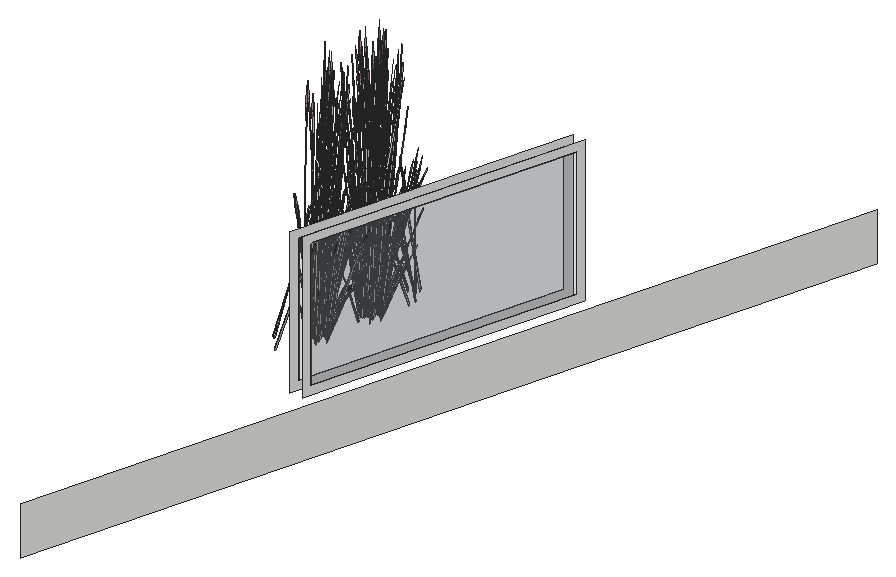
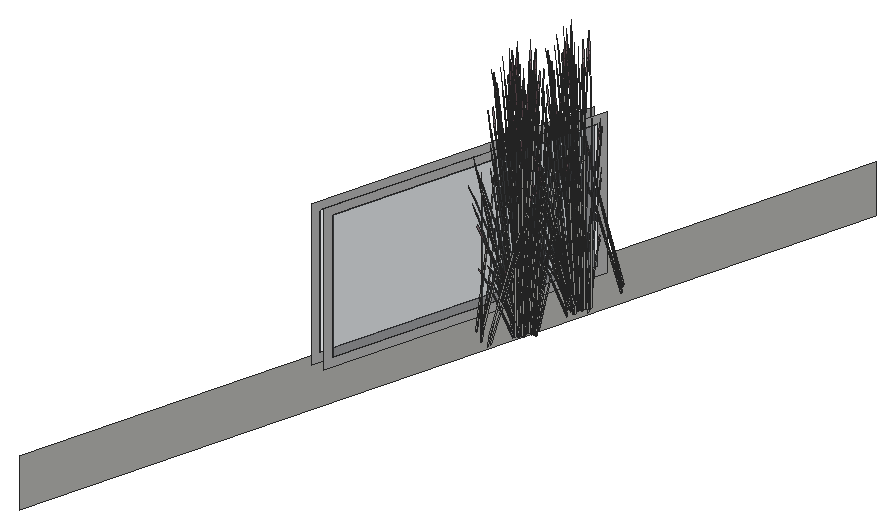
# SketchUp Ruby script. Lengths in inches.
U = 1.inch
M = Sketchup.active_model
def pt(a) = Geom::Point3d.new(a.map { |v| v * U })
def face(e, loops, mat)
  f = e.add_face(loops[0].map { |a| pt(a) })
  loops[1..].each { |l| e.add_face(l.map { |a| pt(a) }).erase! }
  f.material = f.back_material = mat if mat
  f
end
# faces: each face lists its corners as indices into pts; further lists are holes
def faces(e, pts, list, mat = nil) = list.each { |f| face(e, (f[0].is_a?(Array) ? f : [f]).map { |l| l.map { |i| pts[i] } }, mat) }
# xy, xz, yz: faces in a plane at the given z, y or x. An outline is a flat list of corners, or four numbers for a rectangle; further outlines are holes
def ring(l) = l.size == 4 ? [[l[0], l[1]], [l[2], l[1]], [l[2], l[3]], [l[0], l[3]]] : l.each_slice(2).to_a
def flat(e, list, mat, &to3) = list.each { |f| face(e, (f[0].is_a?(Array) ? f : [f]).map { |l| ring(l).map { |u, v| to3.(u, v) } }, mat) }
def xy(e, z, list, mat = nil) = flat(e, list, mat) { |x, y| [x, y, z] }
def xz(e, y, list, mat = nil) = flat(e, list, mat) { |x, z| [x, y, z] }
def yz(e, x, list, mat = nil) = flat(e, list, mat) { |y, z| [x, y, z] }
def lines(e, pts, list) = list.each { |a, b| e.add_line(pt(pts[a]), pt(pts[b])) }
# prism: a flat outline (further loops are holes) pulled along v
def prism(e, loops, v, mat = nil)
  f = face(e, loops, mat); d = Geom::Vector3d.new(v.map { |x| x * U })
  f.pushpull(f.normal.samedirection?(d) ? d.length : -d.length)
end
def box(e, o, s, mat = nil) = prism(e, [[o, [o[0] + s[0], o[1], o[2]], [o[0] + s[0], o[1] + s[1], o[2]], [o[0], o[1] + s[1], o[2]]]], [0, 0, s[2]], mat)
def at(x, y, z, deg = 0) = Geom::Transformation.translation(pt([x, y, z])) * Geom::Transformation.rotation(ORIGIN, Z_AXIS, deg.degrees)
def axes(o, x, y, z) = Geom::Transformation.new([*x, 0, *y, 0, *z, 0, *pt(o).to_a, 1])
def part(name) = M.definitions.add(name)
# library, detail: a bought-in or finely detailed component or shape, given as its bounding box
def library(name, o, s) = part(name).tap { |d| box(d.entities, o, s) }
def detail(e, o, s) = box(e.add_group.entities, o, s)
def put(e, d, t, mat = nil) = e.add_instance(d, t).tap { |i| i.material = mat if mat }
def group(e, t, mat = nil) = e.add_group.tap { |g| g.transformation = t; g.material = mat if mat }.entities
root = M.entities
M.materials.add("Glass_Basic_01").color = [105, 113, 122]
M.materials["Glass_Basic_01"].alpha = 0.25
M.materials.add("LightPink_Translucent").color = [144, 107, 117]
M.materials["LightPink_Translucent"].alpha = 0.75
M.materials.add("M01_Silver_Fog").color = [224, 224, 224]
c1 = part("blade")
p = [[2.15,0.21,22],[0,0.17,0],[0.09,0.45,0],[2.18,0.31,22],[2.29,0.31,22],[0.38,0.45,0],
  [2.48,0.24,33],[2.49,0.24,33],[2.48,0.22,33]]
faces(c1.entities,p,[[0,1,2,3],[4,5,2,3],[6,3,4,7],[8,0,3,6]])
c2 = part("seeds")
p = [[0.3,-0.1,1.38],[-0.01,-0.03,1.59],[-0.01,-0.03,0.03],[0.14,-0.07,-0.07],[0.29,-0.03,3],[0.15,0.01,3.11]]
faces(c2.entities,p,[[0,1,2,3],[1,0,4,5]],"LightPink_Translucent")
c3 = part("blade with seeds")
put(c3.entities,c1,at(0,0,0))
put(c3.entities,c2,axes([2.4,0.25,30.99],[1.5799,-0.05474,1.17369],[-0.12525,1.92788,0.29478],[-0.07173,-0.02425,1.56792]))
p = [[364.95,435.42,522],[307.76,240,522],[307.76,240,510.01],[307.76,240,510],[364.95,435.42,510],[321.22,307.35,558],
  [340.07,371.78,558],[340.07,371.78,522],[321.22,307.35,522],[339.51,369.86,524],[339.51,369.86,556],[321.78,309.27,556],
  [321.78,309.27,524],[343.2,371.78,558],[324.34,307.35,558],[324.34,307.35,522],[343.2,371.78,522],[324.9,309.27,524],
  [324.9,309.27,556],[342.64,369.86,556],[342.64,369.86,524]]
faces(root,p,[[0,1,2,3,4]])
faces(root,p,[[[5,6,7,8],[9,10,11,12]],[[13,14,15,16],[17,18,19,20]]],"M01_Silver_Fog")
faces(root,p,[[10,9,12,11],[18,17,20,19]],"Glass_Basic_01")
put(root,c3,axes([312.83,325.4,524.43],[0.56613,0.26102,0.24065],[-0.27246,0.54236,0.50002],[0,-0.12502,1.60543]))
put(root,c3,axes([313.73,325.53,524.29],[0,0.62282,-0.05637],[-0.62828,0,0],[0,0.01957,1.79368]))
put(root,c3,axes([310.27,315.96,526.53],[0.28589,0.33718,-0.35414],[-0.32644,0.31919,0.4572],[0.16586,0.04856,0.87481]))
put(root,c3,axes([312.65,325.04,524.72],[-0.54562,0.03324,0.44739],[-0.04934,-0.55185,-0.21531],[0.09768,-0.05593,1.43643]))
put(root,c3,axes([314.99,340.47,524.48],[0.47024,0.26927,0.49651],[-0.28107,0.48284,0],[-0.1071,-0.06133,1.57504]))
put(root,c3,axes([312.4,324.09,524.47],[-0.14515,0.53522,0.17642],[-0.53115,-0.15146,0.35086],[0.09175,-0.00261,1.60407]))
put(root,c3,axes([313.43,326.74,524.29],[0.21845,0.61869,-0.06012],[-0.62418,0.21679,0],[0.00763,0.02161,1.72173]))
put(root,c3,axes([315.4375,339.49,524.4375],[0.13317,-0.63814,-0.23429],[0.63143,0.11124,0.51271],[-0.11033,-0.08813,1.5644]))
put(root,c3,axes([315.67,339.64,524.62],[-0.09693,0.48062,0.1448],[-0.47357,-0.08343,-0.41347],[-0.08619,-0.04935,1.26744]))
put(root,c3,axes([316.61,340.98,524.02],[-0.47024,0.26927,-0.49651],[-0.28107,-0.48284,0],[-0.1071,0.06133,1.57504]))
put(root,c3,axes([313.82,338.29,524.02],[0,-0.53854,-0.49651],[0.56215,0,0],[0,-0.12266,1.57504]))
put(root,c3,axes([314.07,338.79,524.48],[0,0.53854,0.49651],[-0.56215,0,0],[0,-0.12266,1.57504]))
put(root,c3,axes([316.64,340.83,524.19],[-0.31023,-0.54153,-0.05142],[0.52557,-0.30095,0.51607],[-0.12951,0.05156,1.6363]))
put(root,c3,axes([312.14,323.43,524.375],[-0.31414,-0.53965,0],[0.52557,-0.30095,-0.51607],[0.1197,-0.06854,1.63711]))
put(root,c3,axes([312.71,327.49,526.98],[0.23981,0.43789,-0.71045],[-0.49365,0.24404,0.08574],[0.05608,0.21158,1.00501]))
put(root,c3,axes([315.24,325.93,524.2],[-0.62797,-0.00431,-0.04976],[0,-0.6019,0.49943],[-0.01973,0.13702,1.58352]))
put(root,c3,axes([314,324.12,524.47],[-0.53992,0.14294,0.17642],[-0.13332,-0.53195,0.35086],[0.04815,0.07751,1.60407]))
put(root,c3,axes([316.5,340.76,524.03],[-0.46876,-0.13325,-0.30978],[0.11803,-0.46926,0.30978],[-0.0945,0.05411,1.38974]))
put(root,c3,axes([313.45,322.125,524.77],[0.06446,0.31404,1.1486],[-0.35756,-0.17393,0.84392],[0.03848,-0.1608,0.25299]))
put(root,c3,axes([315.29,338.92,524.67],[-0.56585,-0.25696,-0.29095],[0.27246,-0.54236,-0.50002],[-0.01778,-0.13316,1.59708]))
put(root,c3,axes([316.77,338.76,524.84],[-0.01373,-0.50706,1.41272],[0.62119,0.13144,0.59816],[-0.14692,0.27746,1.3335]))
put(root,c3,axes([313.12,324.89,524.36],[-0.4166,0.48873,0.45755],[-0.49494,-0.43142,0.17955],[0.10044,-0.04877,1.58856]))
put(root,c3,axes([313.83,325.66,524.21],[0.35073,0.34786,0],[-0.35073,0.34786,0],[0,0,1.69266]))
put(root,c3,axes([313.83,325.26,524.72],[0.24378,-0.48527,0.44739],[0.50654,0.23354,-0.21531],[0,0.11186,1.43643]))
put(root,c3,axes([313.62,326.94,524.2],[0.50654,0.24178,0],[-0.24378,0.50239,0],[0,0,1.74954]))
put(root,c3,axes([312.89,327.58,526.68],[0.49392,0.135,-0.51099],[-0.1693,0.46287,-0.3958],[0.04529,0.18636,0.97773]))
put(root,c3,axes([316.42,339.4,524.67],[0.05855,0.61451,-0.29095],[-0.60981,0.03716,-0.50002],[-0.10738,0.08185,1.59708]))
put(root,c3,axes([315.04,338.37,524.1],[-0.20635,-0.55225,-0.69835],[0.59439,-0.19889,-0.18329],[-0.02281,-0.18701,1.54149]))
put(root,c3,axes([313.66,325.14,524.38],[-0.63506,-0.11347,0.49198],[0.12924,-0.64083,0.19306],[0.09281,0.06188,1.70813]))
put(root,c3,axes([315.97,336.64,526.68],[-0.49392,-0.135,-0.51099],[0.1693,-0.46287,-0.3958],[-0.04529,-0.18636,0.97773]))
put(root,c3,axes([315.11,326.02,524.03],[-0.35073,0.33601,-0.30978],[-0.35073,-0.33601,0.30978],[0,0.10823,1.38974]))
put(root,c3,axes([309.97,315.74,526.98],[0.50227,0.01297,-0.71045],[-0.03373,0.54602,0.08574],[0.21278,0.05762,1.00501]))
put(root,c3,axes([314.11,325.95,524.09],[0.18424,0.49308,-0.69212],[-0.53071,0.17758,-0.18165],[0.02036,0.16697,1.52773]))
put(root,c3,axes([314.07,338.3,524.03],[0.35073,-0.33601,-0.30978],[0.35073,0.33601,0.30978],[0,-0.10823,1.38974]))
put(root,c3,axes([313.85,325.42,524.21],[0.56215,0,0],[0,0.55754,0],[0,0,1.78407]))
put(root,c3,axes([315.65,336.13,524.13],[-0.34721,0.30895,-0.03893],[-0.31814,-0.33837,-0.17649],[-0.0224,-0.09588,0.58215]))
put(root,c3,axes([315.51,339.18,524.36],[0.63506,0.11347,0.45755],[-0.12924,0.64083,0.17955],[-0.09281,-0.06188,1.58856]))
put(root,c3,axes([313.3,324.81,524.72],[-0.30184,-0.45202,0.44739],[0.45719,-0.31831,-0.21531],[0.09768,0.05593,1.43643]))
put(root,c3,axes([312.76,324.92,524.67],[-0.05855,-0.61451,-0.29095],[0.60981,-0.03716,-0.50002],[0.10738,-0.08185,1.59708]))
put(root,c3,axes([314.04,325.37,524.62],[0.46814,-0.15705,0.1448],[0.16394,0.44848,-0.41347],[0,0.0987,1.26744]))
put(root,c3,axes([314.22,323.63,526.68],[-0.35968,-0.36185,-0.51099],[0.37996,-0.3169,-0.3958],[0.05473,-0.18385,0.97773]))
put(root,c3,axes([315.35,339.0625,524.72],[-0.24378,0.48527,0.44739],[-0.50654,-0.23354,-0.21531],[0,-0.11186,1.43643]))
put(root,c3,axes([316.15,336.72,526.98],[-0.23981,-0.43789,-0.71045],[0.49365,-0.24404,0.08574],[-0.05608,-0.21158,1.00501]))
put(root,c3,axes([313.88,325.4,524.67],[0.56585,0.25696,-0.29095],[-0.27246,0.54236,-0.50002],[0.01778,0.13316,1.59708]))
put(root,c3,axes([312.67,323.56,524.03],[0.46876,0.13325,-0.30978],[-0.11803,0.46926,0.30978],[0.0945,-0.05411,1.38974]))
put(root,c3,axes([315.17,340.2,524.47],[0.53992,-0.14294,0.17642],[0.13332,0.53195,0.35086],[-0.04815,-0.07751,1.60407]))
put(root,c3,axes([313.98,322.99,524.59],[-0.14282,0.10901,1.43002],[-0.42773,-0.19079,-0.30754],[0.07929,-0.23728,0.61141]))
put(root,c3,axes([315.86,340.29,524.2],[-0.50654,-0.24178,0],[0.24378,-0.50239,0],[0,0,1.62707]))
put(root,c3,axes([317.04,340.89,524.375],[0.31414,0.53965,0],[-0.52557,0.30095,-0.51607],[-0.1197,0.06854,1.63711]))
put(root,c3,axes([315.11,325.53,524.48],[0,-0.53854,0.49651],[0.56215,0,0],[0,0.12266,1.57504]))
put(root,c3,axes([315.35,326.03,524.02],[0,0.53854,-0.49651],[-0.56215,0,0],[0,0.12266,1.57504]))
put(root,c3,axes([312.56,323.34,524.02],[0.47024,-0.26927,-0.49651],[0.28107,0.48284,0],[0.1071,-0.06133,1.57504]))
put(root,c3,axes([313.17,326.63,525.875],[-0.11485,-0.17291,1.71376],[0.53072,-0.14557,0.13857],[0.11995,0.27145,0.73262]))
put(root,c3,axes([313.51,324.68,524.62],[0.09693,-0.48062,0.1448],[0.47357,0.08343,-0.41347],[0.08619,0.04935,1.26744]))
put(root,c3,axes([311.08,315.47,524.59],[-0.12101,-0.13245,1.43002],[0.15744,-0.43816,-0.30754],[0.24483,0.05936,0.61141]))
put(root,c3,axes([316.78,340.23,524.47],[0.14515,-0.53522,0.17642],[0.53115,0.15146,0.35086],[-0.09175,0.00261,1.60407]))
put(root,c3,axes([316.53,339.52,524.62],[0.37121,0.32357,0.1448],[-0.30963,0.36505,-0.41347],[-0.08619,0.04935,1.26744]))
put(root,c3,axes([314.18,323.85,524.48],[-0.47024,-0.26927,0.49651],[0.28107,-0.48284,0],[0.1071,0.06133,1.57504]))
put(root,c3,axes([314.33,323.8,526.98],[0.01307,-0.49815,-0.71045],[0.55054,0.03346,0.08574],[0.0581,-0.21104,1.00501]))
put(root,c3,axes([316.4,339.12,524.3],[-0.46736,-0.46353,-0.06131],[0.46764,-0.46381,0],[-0.01632,-0.01619,1.75571]))
put(root,c3,axes([316.52,339.28,524.72],[0.54562,-0.03324,0.44739],[0.04934,0.55185,-0.21531],[-0.09768,0.05593,1.43643]))
put(root,c3,axes([313.77,326.66,524.18],[0.5275,-0.18273,-0.19198],[0.18536,0.52636,0.00008],[0.05823,-0.0202,1.73897]))
put(root,c3,axes([316.65,340.55,524.33],[0.62903,0.17504,0.30756],[-0.15737,0.62568,-0.36492],[-0.10411,0.07831,1.64885]))
put(root,c3,axes([315.74,335.75,523.49],[-0.08428,0.0194,1.76342],[-0.46606,-0.21841,-0.26939],[0.00782,-0.18218,0.30037]))
put(root,c3,axes([316.92,340.52,524.48],[0.47024,-0.26927,0.49651],[0.28107,0.48284,0],[-0.1071,0.06133,1.57504]))
put(root,c3,axes([316.2,336.35,526.53],[0.15148,-0.41415,-0.35414],[0.44193,0.12079,0.4572],[-0.04052,-0.16674,0.87481]))
put(root,c3,axes([315.45,338.59,524.36],[0.21845,0.6022,0.45755],[-0.62418,0.20941,0.17955],[0.00763,-0.11065,1.58856]))
put(root,c3,axes([315.35,338.51,524.21],[0.24378,-0.48527,-0.44739],[0.50654,0.23354,0.21531],[0,-0.11186,1.43643]))
put(root,c3,axes([315.98,340.08,524.2],[-0.16394,-0.4643,0],[0.46814,-0.1626,0],[0,0,1.54371]))
put(root,c3,axes([313.78,325.09,524.21],[0.30184,0.45202,-0.44739],[-0.45719,0.31831,0.21531],[0.09768,0.05593,1.43643]))
put(root,c3,axes([314.55,323.5,526.53],[0.33997,-0.28354,-0.35414],[0.32182,0.32376,0.4572],[0.04897,-0.1645,0.87481]))
put(root,c3,axes([314.63,327.14,524.77],[-0.2829,-0.15485,1.1486],[0.36529,-0.15734,0.84392],[0.09853,0.13328,0.25299]))
put(root,c3,axes([313.63,326.98,524.59],[0.00887,-0.17852,1.43002],[0.42372,-0.19941,-0.30754],[0.1308,0.21367,0.61141]))
put(root,c3,axes([313.12,324.45,524.06],[0.33843,-0.40479,-0.62353],[0.42041,0.36705,-0.16365],[0.13561,-0.10098,1.37633]))
put(root,c3,axes([316.64,339.16,524.21],[-0.24378,0.48527,-0.44739],[-0.50654,-0.23354,0.21531],[0,0.11186,1.43643]))
put(root,c3,axes([318.26,347.2,524.59],[-0.03043,0.17617,1.43002],[-0.4448,0.14748,-0.30754],[-0.10397,-0.22771,0.61141]))
put(root,c3,axes([318.41,347.66,525.875],[0.11485,0.17291,1.71376],[-0.53072,0.14557,0.13857],[-0.11995,-0.27145,0.73262]))
put(root,c3,axes([317.6,338.87,524.47],[-0.39477,-0.39228,0.17642],[0.39783,-0.38049,0.35086],[-0.0436,0.08011,1.60407]))
put(root,c3,axes([316.24,338.64,524.21],[0,-0.62313,0],[0.62828,0,0],[0,0,1.79456]))
put(root,c3,axes([314.61,324.09,524.03],[0.11803,0.46926,-0.30978],[-0.46876,0.13325,0.30978],[0.0945,0.05411,1.38974]))
put(root,c3,axes([315.49,325.62,524.375],[0.62828,0,0],[0,0.6019,-0.51607],[0,0.13709,1.63711]))
put(root,c3,axes([315.66,338.75,524.43],[0.56613,0.26102,0.24065],[-0.27246,0.54236,0.50002],[0,-0.12502,1.60543]))
put(root,c3,axes([316.56,338.89,524.29],[0,0.62282,-0.05637],[-0.62828,0,0],[0,0.01957,1.79368]))
put(root,c3,axes([315.47,338.39,524.72],[-0.54562,0.03324,0.44739],[-0.04934,-0.55185,-0.21531],[0.09768,-0.05593,1.43643]))
put(root,c3,axes([313.46,324.84,524.67],[0.5073,-0.35754,-0.29095],[0.33735,0.5052,-0.50002],[0.12516,0.05131,1.59708]))
put(root,c3,axes([315.22,337.44,524.47],[-0.14515,0.53522,0.17642],[-0.53115,-0.15146,0.35086],[0.09175,-0.00261,1.60407]))
put(root,c3,axes([314.68,327.85,524.67],[-0.3222,-0.01689,1.0506],[0.21278,-0.35872,0.58006],[0.12729,0.12745,0.8241]))
put(root,c3,axes([316.26,340.09,524.29],[0.21845,0.61869,-0.06012],[-0.62418,0.21679,0],[0.00763,0.02161,1.72173]))
put(root,c3,axes([313.71,323.55,525.875],[-0.09355,0.18511,1.71376],[-0.39247,-0.38307,0.13857],[0.17705,-0.23875,0.73262]))
put(root,c3,axes([314.96,336.78,524.375],[-0.31414,-0.53965,0],[0.52557,-0.30095,-0.51607],[0.1197,-0.06854,1.63711]))
put(root,c3,axes([318.06,339.28,524.2],[-0.62797,-0.00431,-0.04976],[0,-0.6019,0.49943],[-0.01973,0.13702,1.58352]))
put(root,c3,axes([316.83,337.47,524.47],[-0.53992,0.14294,0.17642],[-0.13332,-0.53195,0.35086],[0.04815,0.07751,1.60407]))
put(root,c3,axes([312.18,324.52,523.59],[-0.49456,0.21561,1.28929],[-0.15741,-0.61865,0.50096],[0.30369,0.01029,1.46642]))
put(root,c3,axes([316.28,335.48,524.77],[0.06446,0.31404,1.1486],[-0.35756,-0.17393,0.84392],[0.03848,-0.1608,0.25299]))
put(root,c3,axes([315.94,338.25,524.36],[-0.4166,0.48873,0.45755],[-0.49494,-0.43142,0.17955],[0.10044,-0.04877,1.58856]))
put(root,c3,axes([316.65,339.02,524.21],[0.35073,0.34786,0],[-0.35073,0.34786,0],[0,0,1.69266]))
put(root,c3,axes([316.65,338.61,524.72],[0.24378,-0.48527,0.44739],[0.50654,0.23354,-0.21531],[0,0.11186,1.43643]))
put(root,c3,axes([316.4375,340.3,524.2],[0.50654,0.24178,0],[-0.24378,0.50239,0],[0,0,1.74954]))
put(root,c3,axes([314,327.36,526.68],[0.4958,-0.12802,-0.51099],[0.08673,0.48481,-0.3958],[0.13317,0.13893,0.97773]))
put(root,c3,axes([314.45,323.5625,524.375],[0.31414,-0.53965,0],[0.52557,0.30095,-0.51607],[0.1197,0.06854,1.63711]))
put(root,c3,axes([314.98,323.33,523.49],[-0.0752,-0.04243,1.76342],[-0.19317,-0.47398,-0.26939],[0.13031,-0.12863,0.30037]))
put(root,c3,axes([316.49,338.49,524.38],[-0.63506,-0.11347,0.49198],[0.12924,-0.64083,0.19306],[0.09281,0.06188,1.70813]))
put(root,c3,axes([314.74,323.89,524.02],[0.47024,0.26927,-0.49651],[-0.28107,0.48284,0],[0.1071,0.06133,1.57504]))
put(root,c3,axes([317.93,339.37,524.03],[-0.35073,0.33601,-0.30978],[-0.35073,-0.33601,0.30978],[0,0.10823,1.38974]))
put(root,c3,axes([314.71,327.72,523.49],[0.03661,-0.07775,1.76342],[0.46087,-0.22898,-0.26939],[0.13972,0.11851,0.30037]))
put(root,c3,axes([314.96,324.47,526.68],[-0.12908,-0.49174,-0.51099],[0.48882,-0.08602,-0.3958],[0.14008,-0.13208,0.97773]))
put(root,c3,axes([316.93,339.31,524.09],[0.18424,0.49308,-0.69212],[-0.53071,0.17758,-0.18165],[0.02036,0.16697,1.52773]))
put(root,c3,axes([316.67,338.78,524.21],[0.56215,0,0],[0,0.55754,0],[0,0,1.78407]))
put(root,c3,axes([315.82,327,525.93],[-0.09617,-0.45271,-0.03492],[0.45453,-0.10408,-0.15832],[0.09492,0.0287,0.52218]))
put(root,c3,axes([316.125,338.16,524.72],[-0.30184,-0.45202,0.44739],[0.45719,-0.31831,-0.21531],[0.09768,0.05593,1.43643]))
put(root,c3,axes([315.58,338.27,524.67],[-0.05855,-0.61451,-0.29095],[0.60981,-0.03716,-0.50002],[0.10738,-0.08185,1.59708]))
put(root,c3,axes([316.86,338.72,524.62],[0.46814,-0.15705,0.1448],[0.16394,0.44848,-0.41347],[0,0.0987,1.26744]))
put(root,c3,axes([317.04,336.99,526.68],[-0.35968,-0.36185,-0.51099],[0.37996,-0.3169,-0.3958],[0.05473,-0.18385,0.97773]))
put(root,c3,axes([314.05,324.92,524.06],[0.52267,0.08829,-0.62353],[-0.11029,0.54463,-0.16365],[0.15598,0.06599,1.37633]))
put(root,c3,axes([316.28,325.24,524.26],[-0.31151,-0.34437,-0.06488],[0.34117,-0.31553,-0.29416],[0.09667,-0.02221,0.97024]))
put(root,c3,axes([316.7,338.76,524.67],[0.56585,0.25696,-0.29095],[-0.27246,0.54236,-0.50002],[0.01778,0.13316,1.59708]))
put(root,c3,axes([315.5625,323.49,524.77],[-0.16736,0.27414,1.1486],[-0.14385,-0.36832,0.84392],[0.13822,-0.09229,0.25299]))
put(root,c3,axes([315.5,336.91,524.03],[0.46876,0.13325,-0.30978],[-0.11803,0.46926,0.30978],[0.0945,-0.05411,1.38974]))
put(root,c3,axes([316.8,336.35,524.59],[-0.14282,0.10901,1.43002],[-0.42773,-0.19079,-0.30754],[0.07929,-0.23728,0.61141]))
put(root,c3,axes([317.93,338.88,524.48],[0,-0.53854,0.49651],[0.56215,0,0],[0,0.12266,1.57504]))
put(root,c3,axes([318.17,339.38,524.02],[0,0.53854,-0.49651],[-0.56215,0,0],[0,0.12266,1.57504]))
put(root,c3,axes([315.39,336.7,524.02],[0.47024,-0.26927,-0.49651],[0.28107,0.48284,0],[0.1071,-0.06133,1.57504]))
put(root,c3,axes([313.94,326.09,525.875],[-0.18664,-0.09279,1.71376],[0.38624,-0.38925,0.13857],[0.24072,0.1756,0.73262]))
put(root,c3,axes([316.33,338.04,524.62],[0.09693,-0.48062,0.1448],[0.47357,0.08343,-0.41347],[0.08619,0.04935,1.26744]))
put(root,c3,axes([315.32,324.52,526.53],[0.43736,-0.07697,-0.35414],[0.11549,0.43998,0.4572],[0.12533,-0.11818,0.87481]))
put(root,c3,axes([314.98,324.67,526.98],[0.26246,-0.42493,-0.71045],[0.45991,0.30199,0.08574],[0.15671,-0.15395,1.00501]))
put(root,c3,axes([314.97,326.95,526.53],[0.28589,0.33718,-0.35414],[-0.32644,0.31919,0.4572],[0.16586,0.04856,0.87481]))
put(root,c3,axes([317,337.2,524.48],[-0.47024,-0.26927,0.49651],[0.28107,-0.48284,0],[0.1071,0.06133,1.57504]))
put(root,c3,axes([317.15,337.15,526.98],[0.01307,-0.49815,-0.71045],[0.55054,0.03346,0.08574],[0.0581,-0.21104,1.00501]))
put(root,c3,axes([316.59,340.01,524.18],[0.5275,-0.18273,-0.19198],[0.18536,0.52636,0.00008],[0.05823,-0.0202,1.73897]))
put(root,c3,axes([319.82,347.79,526.98],[-0.23981,-0.43789,-0.71045],[0.49365,-0.24404,0.08574],[-0.05608,-0.21158,1.00501]))
put(root,c3,axes([316.6,338.45,524.21],[0.30184,0.45202,-0.44739],[-0.45719,0.31831,0.21531],[0.09768,0.05593,1.43643]))
put(root,c3,axes([317.375,336.85,526.53],[0.33997,-0.28354,-0.35414],[0.32182,0.32376,0.4572],[0.04897,-0.1645,0.87481]))
put(root,c3,axes([315.1875,325.56,526.68],[0.13612,-0.48987,-0.51099],[0.46669,0.16791,-0.3958],[0.1879,-0.04492,0.97773]))
put(root,c3,axes([317.46,340.5,524.77],[-0.2829,-0.15485,1.1486],[0.36529,-0.15734,0.84392],[0.09853,0.13328,0.25299]))
put(root,c3,axes([316.45,340.33,524.59],[0.00887,-0.17852,1.43002],[0.42372,-0.19941,-0.30754],[0.1308,0.21367,0.61141]))
put(root,c3,axes([316.36,325.87,524.77],[-0.31044,0.08891,1.1486],[0.14613,-0.36744,0.84392],[0.16469,0.02514,0.25299]))
put(root,c3,axes([315.94,337.8,524.06],[0.33843,-0.40479,-0.62353],[0.42041,0.36705,-0.16365],[0.13561,-0.10098,1.37633]))
put(root,c3,axes([315.36,324.27,524.59],[-0.1795,-0.01595,1.43002],[-0.18389,-0.42791,-0.30754],[0.22051,-0.12105,0.61141]))
put(root,c3,axes([315.48,325.78,526.53],[0.41757,0.15024,-0.35414],[-0.12179,0.4383,0.4572],[0.16812,-0.04019,0.87481]))
put(root,c3,axes([317.43,337.44,524.03],[0.11803,0.46926,-0.30978],[-0.46876,0.13325,0.30978],[0.0945,0.05411,1.38974]))
put(root,c3,axes([318.3125,338.97,524.375],[0.62828,0,0],[0,0.6019,-0.51607],[0,0.13709,1.63711]))
put(root,c3,axes([314.67,326.73,526.98],[0.50227,0.01297,-0.71045],[-0.03373,0.54602,0.08574],[0.21278,0.05762,1.00501]))
put(root,c3,axes([315.6875,325.7,523.98],[-0.32361,0.06463,1.41583],[-0.05151,-0.51444,0.08104],[0.22666,-0.07786,0.80566]))
put(root,c3,axes([319.41,346.82,523.49],[-0.08428,0.0194,1.76342],[-0.46606,-0.21841,-0.26939],[0.00782,-0.18218,0.30037]))
put(root,c3,axes([316.28,338.19,524.67],[0.5073,-0.35754,-0.29095],[0.33735,0.5052,-0.50002],[0.12516,0.05131,1.59708]))
put(root,c3,axes([316.04,325.36,523.49],[-0.02626,-0.08176,1.76342],[0.18213,-0.47826,-0.26939],[0.18372,-0.00688,0.30037]))
put(root,c3,axes([317.5,341.2,524.67],[-0.3222,-0.01689,1.0506],[0.21278,-0.35872,0.58006],[0.12729,0.12745,0.8241]))
put(root,c3,axes([314.34,325.24,525.875],[-0.20841,0.0122,1.71376],[0.13825,-0.52864,0.13857],[0.297,0.0327,0.73262]))
put(root,c3,axes([319.87,347.42,526.53],[0.15148,-0.41415,-0.35414],[0.44193,0.12079,0.4572],[-0.04052,-0.16674,0.87481]))
put(root,c3,axes([316.53,336.9,525.875],[-0.09355,0.18511,1.71376],[-0.39247,-0.38307,0.13857],[0.17705,-0.23875,0.73262]))
put(root,c3,axes([315.1,325.74,526.98],[0.44151,-0.23785,-0.71045],[0.24605,0.4896,0.08574],[0.21333,-0.05562,1.00501]))
put(root,c3,axes([315,337.875,523.59],[-0.49456,0.21561,1.28929],[-0.15741,-0.61865,0.50096],[0.30369,0.01029,1.46642]))
put(root,c3,axes([316.82,340.71,526.68],[0.4958,-0.12802,-0.51099],[0.08673,0.48481,-0.3958],[0.13317,0.13893,0.97773]))
put(root,c3,axes([317.27,336.92,524.375],[0.31414,-0.53965,0],[0.52557,0.30095,-0.51607],[0.1197,0.06854,1.63711]))
put(root,c3,axes([317.8,336.68,523.49],[-0.0752,-0.04243,1.76342],[-0.19317,-0.47398,-0.26939],[0.13031,-0.12863,0.30037]))
put(root,c3,axes([315.78,326.46,524.59],[-0.12101,-0.13245,1.43002],[0.15744,-0.43816,-0.30754],[0.24483,0.05936,0.61141]))
put(root,c3,axes([317.56,337.24,524.02],[0.47024,0.26927,-0.49651],[-0.28107,0.48284,0],[0.1071,0.06133,1.57504]))
put(root,c3,axes([317.54,341.07,523.49],[0.03661,-0.07775,1.76342],[0.46087,-0.22898,-0.26939],[0.13972,0.11851,0.30037]))
put(root,c3,axes([317.78,337.82,526.68],[-0.12908,-0.49174,-0.51099],[0.48882,-0.08602,-0.3958],[0.14008,-0.13208,0.97773]))
put(root,c3,axes([318.64,340.36,525.93],[-0.09617,-0.45271,-0.03492],[0.45453,-0.10408,-0.15832],[0.09492,0.0287,0.52218]))
put(root,c3,axes([316.875,338.27,524.06],[0.52267,0.08829,-0.62353],[-0.11029,0.54463,-0.16365],[0.15598,0.06599,1.37633]))
put(root,c3,axes([319.1,338.59,524.26],[-0.31151,-0.34437,-0.06488],[0.34117,-0.31553,-0.29416],[0.09667,-0.02221,0.97024]))
put(root,c3,axes([318.38,336.84,524.77],[-0.16736,0.27414,1.1486],[-0.14385,-0.36832,0.84392],[0.13822,-0.09229,0.25299]))
put(root,c3,axes([316.77,339.44,525.875],[-0.18664,-0.09279,1.71376],[0.38624,-0.38925,0.13857],[0.24072,0.1756,0.73262]))
put(root,c3,axes([318.14,337.87,526.53],[0.43736,-0.07697,-0.35414],[0.11549,0.43998,0.4572],[0.12533,-0.11818,0.87481]))
put(root,c3,axes([317.8,338.02,526.98],[0.26246,-0.42493,-0.71045],[0.45991,0.30199,0.08574],[0.15671,-0.15395,1.00501]))
put(root,c3,axes([317.79,340.31,526.53],[0.28589,0.33718,-0.35414],[-0.32644,0.31919,0.4572],[0.16586,0.04856,0.87481]))
put(root,c3,axes([320.47,347.41,524.59],[-0.14282,0.10901,1.43002],[-0.42773,-0.19079,-0.30754],[0.07929,-0.23728,0.61141]))
put(root,c3,axes([318.01,338.91,526.68],[0.13612,-0.48987,-0.51099],[0.46669,0.16791,-0.3958],[0.1879,-0.04492,0.97773]))
put(root,c3,axes([319.18,339.22,524.77],[-0.31044,0.08891,1.1486],[0.14613,-0.36744,0.84392],[0.16469,0.02514,0.25299]))
put(root,c3,axes([318.18,337.63,524.59],[-0.1795,-0.01595,1.43002],[-0.18389,-0.42791,-0.30754],[0.22051,-0.12105,0.61141]))
put(root,c3,axes([318.3,339.14,526.53],[0.41757,0.15024,-0.35414],[-0.12179,0.4383,0.4572],[0.16812,-0.04019,0.87481]))
put(root,c3,axes([320.82,348.22,526.98],[0.01307,-0.49815,-0.71045],[0.55054,0.03346,0.08574],[0.0581,-0.21104,1.00501]))
put(root,c3,axes([317.49,340.08,526.98],[0.50227,0.01297,-0.71045],[-0.03373,0.54602,0.08574],[0.21278,0.05762,1.00501]))
put(root,c3,axes([318.51,339.05,523.98],[-0.32361,0.06463,1.41583],[-0.05151,-0.51444,0.08104],[0.22666,-0.07786,0.80566]))
put(root,c3,axes([318.86,338.71,523.49],[-0.02626,-0.08176,1.76342],[0.18213,-0.47826,-0.26939],[0.18372,-0.00688,0.30037]))
put(root,c3,axes([317.16,338.59,525.875],[-0.20841,0.0122,1.71376],[0.13825,-0.52864,0.13857],[0.297,0.0327,0.73262]))
put(root,c3,axes([317.92,339.09,526.98],[0.44151,-0.23785,-0.71045],[0.24605,0.4896,0.08574],[0.21333,-0.05562,1.00501]))
put(root,c3,axes([318.6,339.8125,524.59],[-0.12101,-0.13245,1.43002],[0.15744,-0.43816,-0.30754],[0.24483,0.05936,0.61141]))
put(root,c3,axes([320.2,347.97,525.875],[-0.09355,0.18511,1.71376],[-0.39247,-0.38307,0.13857],[0.17705,-0.23875,0.73262]))
